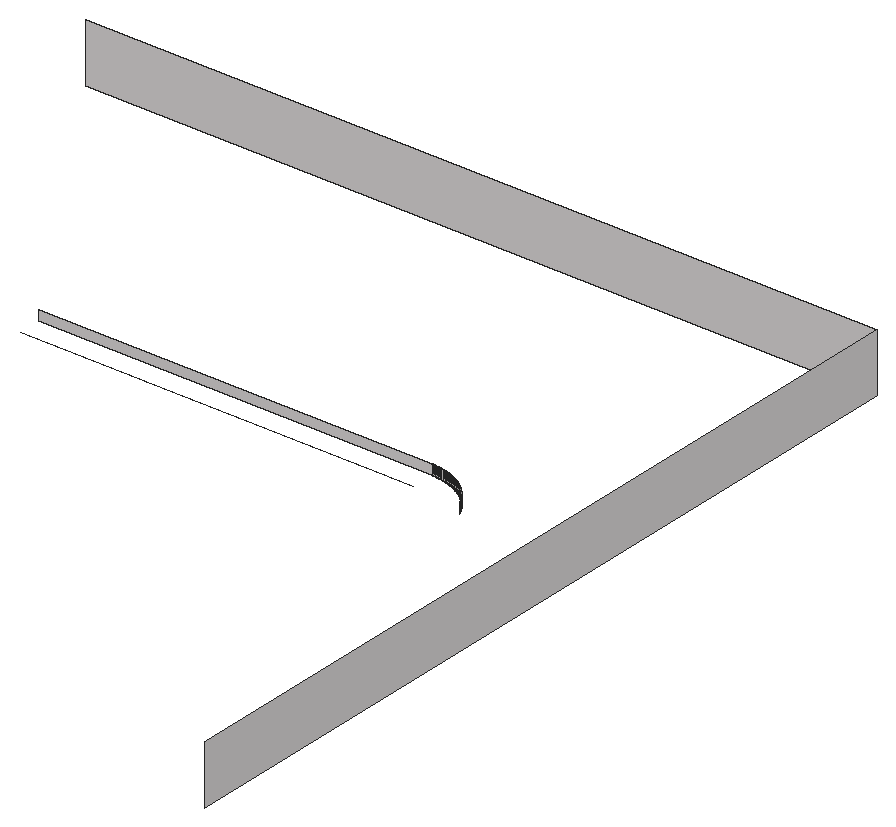
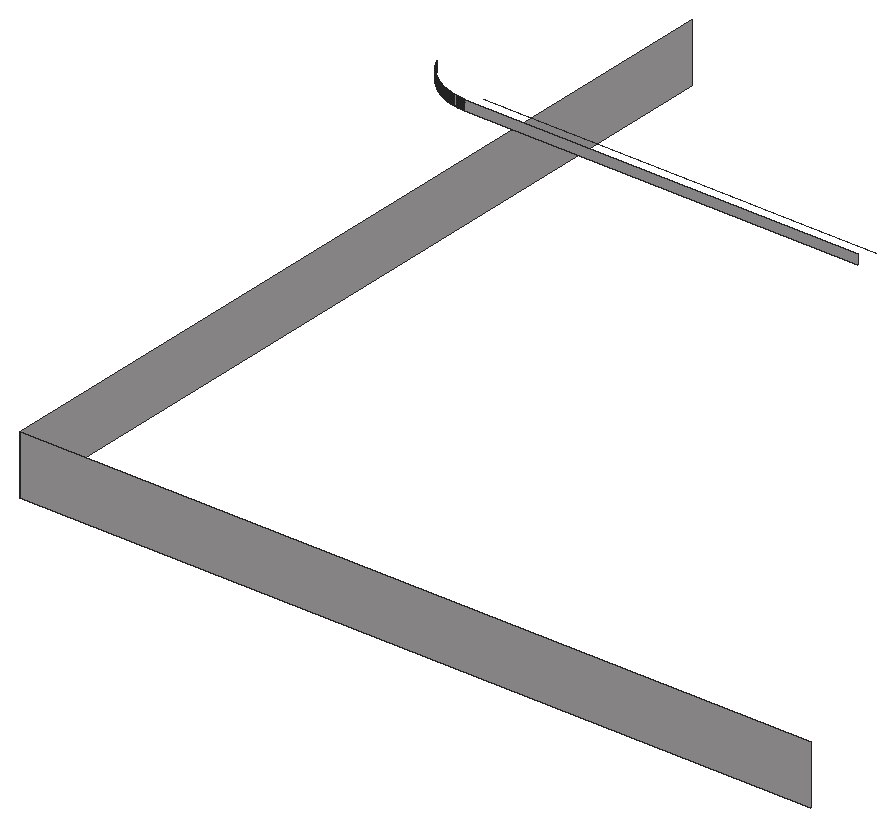
# SketchUp Ruby script. Lengths in inches.
U = 1.inch
M = Sketchup.active_model
def pt(a) = Geom::Point3d.new(a.map { |v| v * U })
def face(e, loops, mat)
  f = e.add_face(loops[0].map { |a| pt(a) })
  loops[1..].each { |l| e.add_face(l.map { |a| pt(a) }).erase! }
  f.material = f.back_material = mat if mat
  f
end
# faces: each face lists its corners as indices into pts; further lists are holes
def faces(e, pts, list, mat = nil) = list.each { |f| face(e, (f[0].is_a?(Array) ? f : [f]).map { |l| l.map { |i| pts[i] } }, mat) }
# xy, xz, yz: faces in a plane at the given z, y or x. An outline is a flat list of corners, or four numbers for a rectangle; further outlines are holes
def ring(l) = l.size == 4 ? [[l[0], l[1]], [l[2], l[1]], [l[2], l[3]], [l[0], l[3]]] : l.each_slice(2).to_a
def flat(e, list, mat, &to3) = list.each { |f| face(e, (f[0].is_a?(Array) ? f : [f]).map { |l| ring(l).map { |u, v| to3.(u, v) } }, mat) }
def xy(e, z, list, mat = nil) = flat(e, list, mat) { |x, y| [x, y, z] }
def xz(e, y, list, mat = nil) = flat(e, list, mat) { |x, z| [x, y, z] }
def yz(e, x, list, mat = nil) = flat(e, list, mat) { |y, z| [x, y, z] }
def lines(e, pts, list) = list.each { |a, b| e.add_line(pt(pts[a]), pt(pts[b])) }
# prism: a flat outline (further loops are holes) pulled along v
def prism(e, loops, v, mat = nil)
  f = face(e, loops, mat); d = Geom::Vector3d.new(v.map { |x| x * U })
  f.pushpull(f.normal.samedirection?(d) ? d.length : -d.length)
end
def box(e, o, s, mat = nil) = prism(e, [[o, [o[0] + s[0], o[1], o[2]], [o[0] + s[0], o[1] + s[1], o[2]], [o[0], o[1] + s[1], o[2]]]], [0, 0, s[2]], mat)
def at(x, y, z, deg = 0) = Geom::Transformation.translation(pt([x, y, z])) * Geom::Transformation.rotation(ORIGIN, Z_AXIS, deg.degrees)
def axes(o, x, y, z) = Geom::Transformation.new([*x, 0, *y, 0, *z, 0, *pt(o).to_a, 1])
def part(name) = M.definitions.add(name)
# library, detail: a bought-in or finely detailed component or shape, given as its bounding box
def library(name, o, s) = part(name).tap { |d| box(d.entities, o, s) }
def detail(e, o, s) = box(e.add_group.entities, o, s)
def put(e, d, t, mat = nil) = e.add_instance(d, t).tap { |i| i.material = mat if mat }
def group(e, t, mat = nil) = e.add_group.tap { |g| g.transformation = t; g.material = mat if mat }.entities
root = M.entities
M.materials.add("[Quartz Light Brown]").color = [215, 212, 212]
xz(root,478.7,[[225,480,464,486],[464,480,464.5,486]],"[Quartz Light Brown]")
xz(root,787,[[7,396,488,432]],"[Quartz Light Brown]")
yz(root,488,[[276.5,396,787,432]],"[Quartz Light Brown]")
p = [[498.08,457.51,480],[497.86,457.95,480],[497.86,457.95,486],[498.08,457.51,486],[497.63,458.39,480],[497.63,458.39,486],
  [497.4,458.83,480],[497.4,458.83,486],[497.15,459.27,480],[497.15,459.27,486],[496.91,459.7,480],[496.91,459.7,486],
  [496.66,460.13,480],[496.66,460.13,486],[496.4,460.56,480],[496.4,460.56,486],[496.14,460.98,480],[496.14,460.98,486],
  [495.87,461.4,480],[495.87,461.4,486],[495.6,461.8125,480],[495.6,461.8125,486],[495.32,462.22,480],[495.32,462.22,486],
  [495.03,462.63,480],[495.03,462.63,486],[494.74,463.04,480],[494.74,463.04,486],[494.45,463.4375,480],[494.45,463.4375,486],
  [494.15,463.83,480],[494.15,463.83,486],[493.84,464.23,480],[493.84,464.23,486],[493.53,464.62,480],[493.53,464.62,486],
  [493.22,465,480],[493.22,465,486],[492.9,465.38,480],[492.9,465.38,486],[492.57,465.76,480],[492.57,465.76,486],
  [492.24,466.13,480],[492.24,466.13,486],[491.9,466.5,480],[491.9,466.5,486],[491.5625,466.86,480],[491.5625,466.86,486],
  [491.22,467.22,480],[491.22,467.22,486],[490.87,467.57,480],[490.87,467.57,486],[490.52,467.92,480],[490.52,467.92,486],
  [490.16,468.27,480],[490.16,468.27,486],[489.79,468.61,480],[489.79,468.61,486],[489.43,468.94,480],[489.43,468.94,486],
  [489.06,469.27,480],[489.06,469.27,486],[488.68,469.6,480],[488.68,469.6,486],[488.3,469.92,480],[488.3,469.92,486],
  [487.91,470.23,480],[487.91,470.23,486],[487.53,470.54,480],[487.53,470.54,486],[487.13,470.85,480],[487.13,470.85,486],
  [486.74,471.15,480],[486.74,471.15,486],[486.34,471.44,480],[486.34,471.44,486],[485.93,471.73,480],[485.93,471.73,486],
  [485.52,472.02,480],[485.52,472.02,486],[485.11,472.3,480],[485.11,472.3,486],[484.7,472.57,480],[484.7,472.57,486],
  [484.28,472.84,480],[484.28,472.84,486],[483.85,473.1,480],[483.85,473.1,486],[483.43,473.36,480],[483.43,473.36,486],
  [483,473.61,480],[483,473.61,486],[482.57,473.86,480],[482.57,473.86,486],[482.13,474.1,480],[482.13,474.1,486],
  [481.69,474.33,480],[481.69,474.33,486],[481.25,474.56,480],[481.25,474.56,486],[480.81,474.78,480],[480.81,474.78,486],
  [480.36,475,480],[480.36,475,486],[479.91,475.21,480],[479.91,475.21,486],[479.46,475.42,480],[479.46,475.42,486],
  [479,475.62,480],[479,475.62,486],[478.54,475.81,480],[478.54,475.81,486],[478.08,476,480],[478.08,476,486],
  [477.62,476.18,480],[477.62,476.18,486],[477.15,476.35,480],[477.15,476.35,486],[476.68,476.52,480],[476.68,476.52,486],
  [476.21,476.68,480],[476.21,476.68,486],[475.74,476.84,480],[475.74,476.84,486],[475.27,476.99,480],[475.27,476.99,486],
  [474.79,477.14,480],[474.79,477.14,486],[474.31,477.27,480],[474.31,477.27,486],[473.84,477.41,480],[473.84,477.41,486],
  [473.35,477.53,480],[473.35,477.53,486],[472.87,477.65,480],[472.87,477.65,486],[472.39,477.76,480],[472.39,477.76,486],
  [471.9,477.87,480],[471.9,477.87,486],[471.41,477.97,480],[471.41,477.97,486],[470.92,478.06,480],[470.92,478.06,486],
  [470.44,478.15,480],[470.44,478.15,486],[469.94,478.23,480],[469.45,478.31,480],[469.45,478.31,486],[469.94,478.23,486],
  [468.96,478.375,480],[468.96,478.375,486],[468.47,478.4375,480],[467.97,478.49,480],[467.97,478.49,486],[468.47,478.4375,486],
  [467.48,478.54,480],[466.98,478.58,480],[466.98,478.58,486],[467.48,478.54,486],[465.99,478.65,480],[465.49,478.67,480],
  [465.49,478.67,486],[465.99,478.65,486],[466.49,478.62,480],[466.49,478.62,486],[464.99,478.6875,480],[464.5,478.7,480],
  [464.5,478.7,486],[464.99,478.6875,486],[225,464.7,480],[464,464.7,480]]
faces(root,p,[[0,1,2,3],[1,4,5,2],[4,6,7,5],[6,8,9,7],[8,10,11,9],[10,12,13,11],[12,14,15,13],[14,16,17,15],
  [16,18,19,17],[18,20,21,19],[20,22,23,21],[22,24,25,23],[24,26,27,25],[26,28,29,27],[28,30,31,29],[30,32,33,31],
  [32,34,35,33],[34,36,37,35],[36,38,39,37],[38,40,41,39],[40,42,43,41],[42,44,45,43],[44,46,47,45],[46,48,49,47],
  [48,50,51,49],[50,52,53,51],[52,54,55,53],[54,56,57,55],[56,58,59,57],[58,60,61,59],[60,62,63,61],[62,64,65,63],
  [64,66,67,65],[66,68,69,67],[68,70,71,69],[70,72,73,71],[72,74,75,73],[74,76,77,75],[76,78,79,77],[78,80,81,79],
  [80,82,83,81],[82,84,85,83],[84,86,87,85],[86,88,89,87],[88,90,91,89],[90,92,93,91],[92,94,95,93],[94,96,97,95],
  [96,98,99,97],[98,100,101,99],[100,102,103,101],[102,104,105,103],[104,106,107,105],[106,108,109,107],[108,110,111,109],[110,112,113,111],
  [112,114,115,113],[114,116,117,115],[116,118,119,117],[118,120,121,119],[120,122,123,121],[122,124,125,123],[124,126,127,125],[126,128,129,127],
  [128,130,131,129],[130,132,133,131],[132,134,135,133],[134,136,137,135],[136,138,139,137],[138,140,141,139],[140,142,143,141],[142,144,145,143],
  [146,147,148,149],[144,146,149,145],[147,150,151,148],[152,153,154,155],[150,152,155,151],[156,157,158,159],[153,156,159,154],[160,161,162,163],
  [164,160,163,165],[157,164,165,158],[166,167,168,169],[161,166,169,162]],"[Quartz Light Brown]")
lines(root,p,[[170,171]])
